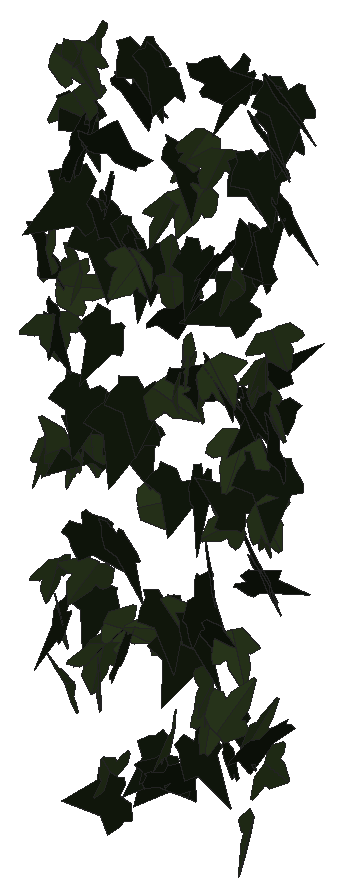
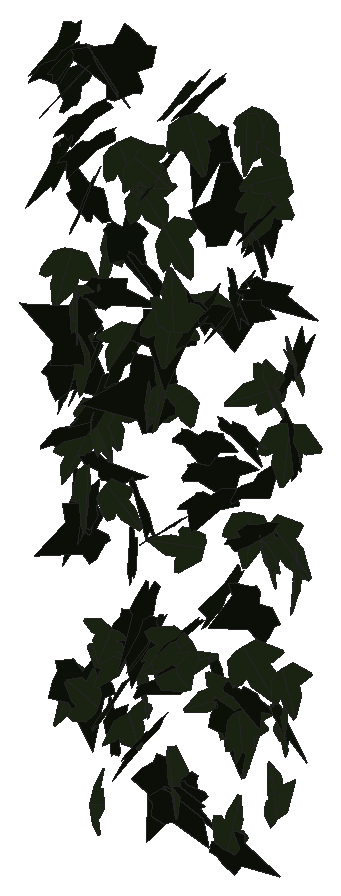
# SketchUp Ruby script. Lengths in inches.
U = 1.inch
M = Sketchup.active_model
def pt(a) = Geom::Point3d.new(a.map { |v| v * U })
def face(e, loops, mat)
  f = e.add_face(loops[0].map { |a| pt(a) })
  loops[1..].each { |l| e.add_face(l.map { |a| pt(a) }).erase! }
  f.material = f.back_material = mat if mat
  f
end
# faces: each face lists its corners as indices into pts; further lists are holes
def faces(e, pts, list, mat = nil) = list.each { |f| face(e, (f[0].is_a?(Array) ? f : [f]).map { |l| l.map { |i| pts[i] } }, mat) }
# xy, xz, yz: faces in a plane at the given z, y or x. An outline is a flat list of corners, or four numbers for a rectangle; further outlines are holes
def ring(l) = l.size == 4 ? [[l[0], l[1]], [l[2], l[1]], [l[2], l[3]], [l[0], l[3]]] : l.each_slice(2).to_a
def flat(e, list, mat, &to3) = list.each { |f| face(e, (f[0].is_a?(Array) ? f : [f]).map { |l| ring(l).map { |u, v| to3.(u, v) } }, mat) }
def xy(e, z, list, mat = nil) = flat(e, list, mat) { |x, y| [x, y, z] }
def xz(e, y, list, mat = nil) = flat(e, list, mat) { |x, z| [x, y, z] }
def yz(e, x, list, mat = nil) = flat(e, list, mat) { |y, z| [x, y, z] }
def lines(e, pts, list) = list.each { |a, b| e.add_line(pt(pts[a]), pt(pts[b])) }
# prism: a flat outline (further loops are holes) pulled along v
def prism(e, loops, v, mat = nil)
  f = face(e, loops, mat); d = Geom::Vector3d.new(v.map { |x| x * U })
  f.pushpull(f.normal.samedirection?(d) ? d.length : -d.length)
end
def box(e, o, s, mat = nil) = prism(e, [[o, [o[0] + s[0], o[1], o[2]], [o[0] + s[0], o[1] + s[1], o[2]], [o[0], o[1] + s[1], o[2]]]], [0, 0, s[2]], mat)
def at(x, y, z, deg = 0) = Geom::Transformation.translation(pt([x, y, z])) * Geom::Transformation.rotation(ORIGIN, Z_AXIS, deg.degrees)
def axes(o, x, y, z) = Geom::Transformation.new([*x, 0, *y, 0, *z, 0, *pt(o).to_a, 1])
def part(name) = M.definitions.add(name)
# library, detail: a bought-in or finely detailed component or shape, given as its bounding box
def library(name, o, s) = part(name).tap { |d| box(d.entities, o, s) }
def detail(e, o, s) = box(e.add_group.entities, o, s)
def put(e, d, t, mat = nil) = e.add_instance(d, t).tap { |i| i.material = mat if mat }
def group(e, t, mat = nil) = e.add_group.tap { |g| g.transformation = t; g.material = mat if mat }.entities
root = M.entities
M.materials.add("efeu1").color = [18, 25, 13]
M.materials.add("efeu2").color = [43, 57, 29]
c1 = part("ivyleaf_9")
p = [[1.54,2.16,1.25],[1.36,2.04,1.19],[-0.21,0.99,0.68],[-0.71,1.11,0.82],[-0.85,0.86,0.67],[-0.8,0.17,0.21],
  [-0.9,-0.01,0.1],[-0.67,-0.16,-0.02],[-0.08,-0.08,-0.05],[-0.03,-0.6,-0.4],[0.65,-0.88,-0.66],[0.83,-0.6,-0.49],
  [1.29,-0.42,-0.43],[1.8125,-0.07,-0.26],[1.21,0.44,0.15]]
faces(c1.entities,p,[[0,1,2,3,4,5,6,7,8,9,10,11,12,13,14]],"efeu1")
c2 = part("ivyleaf_10")
p = [[0,0.5,-0.03],[-0.0625,2.02,-0.43],[-0.19,2.01,-0.46],[-0.54,1.05,-0.29],[-0.52,0.625,-0.18],[-0.83,0.76,-0.28],
  [-1.16,0.64,-0.33],[-1.15,0.33,-0.24],[-0.77,-0.39,0.02],[-0.3,-0.51,0.16],[0.04,-0.48,0.23],[-0.02,2.01,-0.4375],
  [-0.06,2.01,-0.43],[0.04,-0.49,0.23],[0.67,-0.49,0.14],[1.38,0.36,-0.2],[1.375,0.51,-0.24],[0.81,0.65,-0.19],
  [0.62,0.59,-0.15],[0.6,1.09,-0.28],[0.5,1.23,-0.31]]
faces(c2.entities,p,[[0,1,2,3,4,5,6,7,8,9,10],[11,12,0,13,14,15,16,17,18,19,20]],"efeu2")
put(root,c1,axes([556.96,126.85,213.5],[-0.04115,0.46001,0.83642],[-0.11422,0.82881,-0.46144],[-0.94771,-0.11987,0.0193]))
put(root,c2,axes([563.91,127.77,229.87],[0.04295,-0.99561,0.12288],[0.05249,-0.1206,-0.99543],[1.00179,0.049,0.04689]))
put(root,c2,axes([562.57,126.82,212.66],[0.29842,0.56117,-0.90359],[0.36551,0.82723,0.63446],[0.9989,-0.47034,0.03779]))
put(root,c1,axes([563.42,128.23,219.59],[-0.00074,-0.33269,1.07237],[0.43668,-0.98803,-0.30622],[1.0344,0.41687,0.13005]))
put(root,c1,axes([556.12,127.79,206.37],[-0.18509,-0.18046,-0.9132],[-0.73724,-0.54002,0.25614],[-0.56831,0.75932,-0.03487]))
put(root,c2,axes([554.31,127.5,241.82],[-1.02474,0.14394,-0.2906],[0.28612,-0.0521,-1.03473],[-0.15266,-1.06387,0.01136]))
put(root,c2,axes([555.28,127.78,213.03],[-0.45322,-0.9324,0.17488],[-0.04544,-0.17226,-1.03616],[0.94757,-0.45422,0.03396]))
put(root,c1,axes([551.96,128.43,230.85],[-0.09599,-0.54405,0.96814],[0.20635,-0.96357,-0.52102],[1.0912,0.13435,0.18369]))
put(root,c1,axes([558.13,128.39,241.92],[-0.10549,-0.86154,0.61105],[0.18313,-0.6197,-0.84213],[1.04024,0.02173,0.21022]))
put(root,c2,axes([561.73,127.32,229.05],[0.31502,0.84677,0.37219],[0.14771,0.34208,-0.9033],[-0.91309,0.34748,-0.01772]))
put(root,c2,axes([564.7,127.16,211.14],[-0.06467,-0.7813,-0.75993],[0.13916,0.74912,-0.78203],[1.081,-0.14318,0.05521]))
put(root,c2,axes([557.07,127.76,232.33],[0.90924,-0.05206,-0.47628],[-0.4752,0.03248,-0.91072],[0.06118,1.02592,0.00467]))
put(root,c1,axes([563.52,128.48,234.65],[-0.09725,-0.35412,0.97283],[-0.07663,-0.97197,-0.36147],[1.03244,-0.1055,0.0648]))
put(root,c2,axes([558.8,127.46,226.9],[-0.4961,-0.37935,-0.73161],[0.7217,0.21231,-0.59946],[0.39789,-0.85808,0.17512]))
put(root,c1,axes([556.53,128.1875,224.72],[-0.65603,-0.87187,-0.17445],[0.10966,0.1358,-1.0911],[0.88236,-0.6651,0.0059]))
put(root,c2,axes([554.79,128.13,211.92],[0.37628,-0.38277,0.77565],[0.65648,-0.42438,-0.52789],[0.56318,0.75041,0.09711]))
put(root,c1,axes([563.4,127.71,234.61],[-0.44422,0.38361,0.92445],[0.64946,-0.65908,0.58558],[0.76155,0.78584,0.03985]))
put(root,c1,axes([554.09,128.3,224.9],[-0.23015,-0.99245,0.12721],[-0.02988,-0.12366,-1.01878],[1.00012,-0.23208,-0.00116]))
put(root,c2,axes([560.25,128.13,236.59],[-0.45584,-0.70848,0.50873],[-0.08625,-0.53459,-0.82177],[0.86793,-0.42522,0.18553]))
put(root,c2,axes([555.53,128.26,207],[-0.15251,-0.70602,-0.60976],[-0.02381,-0.6147,0.7177],[-0.93258,0.13116,0.08139]))
put(root,c2,axes([553.34,127.74,222.29],[-0.62841,-0.13183,0.94599],[-0.92672,-0.18997,-0.64208],[0.23121,-1.11969,-0.00244]))
put(root,c1,axes([564.24,128.47,225.67],[-0.07422,-0.27151,1.00837],[0.08294,-1.00925,-0.26565],[1.04098,0.06105,0.09306]))
put(root,c1,axes([560.77,128.25,218.3],[-0.03714,0.01892,0.92509],[0.16725,-0.91044,0.02533],[0.91004,0.1681,0.0331]))
put(root,c1,axes([554.34,126.93,237.34],[-0.1579,0.36324,-1.00284],[-0.76071,0.67224,0.36327],[0.74762,0.76073,0.15783]))
put(root,c1,axes([555.83,128.14,218.61],[0.54822,-0.90912,0.265],[0.14478,-0.22214,-1.06159],[0.93583,0.56695,0.009]))
put(root,c1,axes([559.26,128.38,237.93],[0.26468,-0.96173,0.46345],[0.13628,-0.44313,-0.9974],[1.05883,0.29744,0.01253]))
put(root,c1,axes([561.17,128.36,228.1],[0.26521,-0.70377,0.63807],[0.28525,-0.57289,-0.75045],[0.90612,0.38634,0.04949]))
put(root,c1,axes([563.62,128.24,240.77],[0.47323,-0.6754,0.56397],[0.33323,-0.4551,-0.82464],[0.81437,0.5787,0.0097]))
put(root,c1,axes([563.26,127.54,228],[0.72881,-0.37273,-0.58808],[-0.51666,0.28116,-0.8185],[0.46672,0.89328,0.01224]))
put(root,c2,axes([564.69,127.67,231.62],[-0.60628,-0.74749,-0.29267],[0.20858,0.20748,-0.96199],[0.77517,-0.64046,0.02994]))
put(root,c1,axes([561.55,127.875,234.3],[-0.40553,0.79059,-0.42816],[0.18074,-0.38843,-0.88841],[-0.88073,-0.44374,0.01483]))
put(root,c1,axes([563.53,128.13,239.35],[0.05083,-0.96506,-0.23992],[0.00881,0.24066,-0.96617],[0.9944,0.0472,0.02083]))
put(root,c1,axes([557.15,128.1,242.55],[0.28565,-1.0189,-0.20422],[0.00259,0.21249,-1.05655],[1.03917,0.27955,0.05877]))
put(root,c1,axes([553.07,128.06,213.98],[-0.79451,0.38254,-0.44095],[0.40062,-0.18434,-0.88178],[-0.42458,-0.88978,-0.00689]))
put(root,c2,axes([564.125,127.49,222.92],[0.08424,0.91846,0.37096],[0.03967,0.36887,-0.9223],[-0.98976,0.09296,-0.00539]))
put(root,c2,axes([560.96,127.72,213.3],[0.71943,-0.66194,-0.52085],[-0.32633,0.41243,-0.9749],[0.77651,0.78661,0.07286]))
put(root,c2,axes([559.3125,128.41,228.77],[-0.42038,0.24619,-0.83192],[0.34213,-0.80248,-0.41036],[-0.79727,-0.47417,0.26255]))
put(root,c1,axes([553.96,128.42,234.27],[-0.97197,-0.29067,0.36021],[-0.34794,-0.09369,-1.01445],[0.30525,-1.03232,-0.00936]))
put(root,c1,axes([563.79,127.67,219.99],[0.8011,-0.12733,-0.47848],[-0.47631,0.0504,-0.81087],[0.13523,0.93175,-0.02153]))
put(root,c1,axes([555.26,128.25,236.91],[1.16197,0.04712,0.13204],[-0.13204,-0.00281,1.16293],[0.04714,-1.16945,0.00252]))
put(root,c2,axes([564.03,127.77,230.06],[0.27753,-0.94116,-0.40182],[-0.03605,0.40708,-0.97839],[1.02271,0.26975,0.07455]))
put(root,c2,axes([562.48,128.08,225.45],[1.05871,0.30675,-0.19017],[-0.18227,-0.05426,-1.10226],[-0.31151,1.07429,-0.00137]))
put(root,c1,axes([560.25,127.9,210.29],[0.53104,-0.81397,-0.44891],[-0.17305,0.42139,-0.96878],[0.9133,0.55313,0.07746]))
put(root,c1,axes([557.07,128.29,226.02],[-0.60219,-0.61477,-0.41336],[0.31879,0.26581,-0.85974],[0.66872,-0.68032,0.03762]))
put(root,c2,axes([552,127.98,230.5625],[0.8213,-0.66676,0.03168],[-0.00422,0.04505,1.05738],[-0.66749,-0.82067,0.0323]))
put(root,c2,axes([561.95,128.16,221.43],[-0.56678,0.00415,0.74017],[-0.70589,-0.28349,-0.53894],[0.22268,-0.8881,0.17549]))
put(root,c1,axes([554.26,127.9,218.65],[-0.07936,-0.03443,-0.9948],[0.7537,0.64979,-0.08262],[0.6502,-0.75743,-0.02565]))
put(root,c1,axes([563.87,127.72,211.84],[-0.05359,1.11353,-0.19815],[-0.01265,-0.19895,-1.11461],[-1.13096,-0.05054,0.02186]))
put(root,c1,axes([551.9,128.47,227.67],[0.08296,-0.19874,-1.04068],[1.05949,0.01867,0.08089],[0.00316,-1.04382,0.19959]))
put(root,c1,axes([562.7,127.99,222.3],[-0.28638,0.3559,0.81761],[-0.80241,0.27173,-0.39934],[-0.38896,-0.8226,0.22183]))
put(root,c1,axes([557.125,128.48,232.6],[-0.68031,-0.23476,-0.695],[0.70664,0.04481,-0.70683],[0.19698,-0.97152,0.13535]))
put(root,c1,axes([558.13,128.55,215.97],[0.14563,-1.01866,-0.0126],[-0.00212,0.01243,-1.02901],[1.01873,0.14565,-0.00034]))
put(root,c2,axes([562.34,128.82,206.54],[0.23114,-0.45617,0.968],[0.64244,-0.73284,-0.49876],[0.8558,0.67334,0.11297]))
put(root,c1,axes([563.89,128.62,227.57],[-0.09923,0.41129,-0.95314],[0.07181,-0.95247,-0.41847],[-1.0356,-0.10546,0.06231]))
put(root,c1,axes([558.89,127.63,208.53],[0.66064,0.78429,-0.03153],[-0.02649,-0.01891,-1.02542],[-0.78447,0.66112,0.00808]))
put(root,c2,axes([552.36,128.38,215.93],[-0.13703,-0.89487,0.15217],[0.00386,-0.15447,-0.9049],[0.90771,-0.13444,0.02683]))
put(root,c1,axes([560.88,127.97,242.35],[0.52466,-0.06465,0.98926],[0.98462,-0.0964,-0.5285],[0.11549,1.11562,0.01166]))
put(root,c2,axes([554.23,128.51,216.35],[-0.58443,-0.66081,0.51555],[-0.3443,-0.38374,-0.88217],[0.76414,-0.6783,-0.00317]))
put(root,c2,axes([552.05,127.89,221.61],[0.35329,-0.86472,-0.61308],[-0.04541,0.6333,-0.9194],[1.05903,0.31563,0.1651]))
put(root,c2,axes([552.1875,128.64,213.52],[0.19262,-0.27309,0.86289],[0.80434,-0.35283,-0.29121],[0.41496,0.81067,0.16394]))
put(root,c1,axes([558.33,128.4,208.17],[0.20273,0.38091,-0.79878],[-0.3916,-0.69626,-0.43141],[-0.79359,0.44087,0.00882]))
put(root,c2,axes([558.34,128.68,235.43],[-0.01819,-1.0076,0.41582],[-0.03428,-0.41514,-1.00746],[1.08949,-0.02988,-0.02475]))
put(root,c1,axes([559.89,128.62,233.46],[-0.75738,-0.18548,-0.58185],[0.58904,0.02278,-0.77401],[0.16118,-0.9548,0.09457]))
put(root,c2,axes([562.34,127.76,233.52],[0.13966,-0.75749,-0.81498],[-0.06329,0.81464,-0.76802],[1.11085,0.14165,0.05871]))
put(root,c1,axes([563.66,128.75,224.4],[-0.1714,-1.08547,-0.1402],[0.03643,0.13617,-1.09882],[1.09388,-0.17461,0.01463]))
put(root,c2,axes([553.36,128.45,221.91],[0.77331,-0.51798,0.01839],[0.01642,-0.00854,-0.93075],[0.51804,0.77348,0.00205]))
put(root,c1,axes([555.04,128.625,233.08],[-0.4878,-0.88386,-0.4176],[0.17964,0.3777,-1.00927],[0.9609,-0.51931,-0.02331]))
put(root,c1,axes([562.02,128.1,209.67],[0.20362,-0.3916,0.81944],[-0.28081,0.77149,0.43846],[-0.8637,-0.34315,0.05063]))
put(root,c1,axes([556.76,127.97,240.72],[0.88102,0.28104,-0.58194],[-0.56829,-0.13157,-0.92389],[-0.30771,1.04763,0.04009]))
put(root,c2,axes([554.43,128.26,222.69],[-0.91617,-0.23142,0.04825],[-0.04604,-0.01476,-0.94494],[0.23187,-0.91732,0.00303]))
put(root,c1,axes([559.5625,128.62,215.38],[0.56135,-0.8755,0.09688],[0.05414,-0.08038,-1.04001],[0.87918,0.56395,0.00218]))
put(root,c2,axes([561.03,128.6,238.54],[-0.42852,-0.82164,0.33797],[-0.16099,-0.29721,-0.92666],[0.87373,-0.45773,-0.00498]))
put(root,c1,axes([554.13,129,222.53],[-0.66689,-0.54566,0.43347],[-0.30315,-0.31309,-0.8605],[0.62749,-0.73118,0.04497]))
put(root,c2,axes([552.3125,128.29,227.7],[-0.79347,-0.70618,-0.08184],[0.06106,0.05449,-1.06221],[0.70828,-0.79582,-0.00011]))
put(root,c1,axes([563.2,127.84,219.19],[0.7574,0.30109,0.46491],[0.4054,0.23533,-0.81285],[-0.37743,0.85699,0.05987]))
put(root,c2,axes([558.25,129.02,214.58],[0.03717,0.29167,1.04358],[-0.44389,-0.94845,0.28089],[0.98847,-0.43689,0.0869]))
put(root,c1,axes([553.43,128.58,236.01],[-0.10786,0.66897,0.83861],[0.12026,-0.82998,0.67756],[1.06598,0.16133,0.00842]))
put(root,c2,axes([559.46,128.79,226.48],[-0.61943,0.18058,0.88303],[0.81607,-0.34245,0.64249],[0.38259,1.02282,0.05921]))
put(root,c1,axes([557.93,128.71,208.57],[-0.90536,-0.01366,-0.00853],[0.00854,-0.00012,-0.90546],[0.01365,-0.9054,0.00025]))
put(root,c1,axes([556.55,129.19,232],[0.15202,-0.85598,0.74744],[0.2793,-0.70283,-0.86169],[1.10153,0.29633,0.11534]))
put(root,c1,axes([559,128.0625,230.72],[0.2379,0.92417,-0.18748],[-0.0666,-0.1764,-0.95409],[-0.94064,0.24623,0.02014]))
put(root,c2,axes([563.24,128.7,227.95],[-0.67483,0.42661,-0.8087],[0.63847,-0.49959,-0.79633],[-0.65448,-0.92725,0.05699]))
put(root,c1,axes([558.8,129.12,213.95],[-0.37855,-0.89782,0.18594],[-0.04726,-0.18179,-0.974],[0.91566,-0.38056,0.02661]))
put(root,c2,axes([554.43,128.32,242.07],[0.01777,-0.94548,-0.37206],[-0.01894,0.37174,-0.94558],[1.01587,0.02347,-0.01112]))
put(root,c2,axes([559.77,128.9,238.6875],[0.29669,0.72316,-0.64219],[-0.46401,-0.48294,-0.7582],[-0.84857,0.51692,0.19006]))
put(root,c2,axes([552.32,128.99,209.92],[-0.70394,0.04576,0.86687],[0.79463,-0.41533,0.6672],[0.34946,1.03658,0.22906]))
put(root,c2,axes([553.5,128.32,238.92],[-0.52945,-0.8289,-0.45128],[0.25109,0.37508,-0.98352],[0.90977,-0.5859,0.00882]))
put(root,c1,axes([562.1,128.91,242.72],[-0.87324,0.16856,-0.48498],[0.45597,-0.18524,-0.88541],[-0.23601,-0.98155,0.08382]))
put(root,c1,axes([561.99,129.07,231.71],[-0.78993,-0.22021,0.56102],[-0.5372,-0.16203,-0.81999],[0.27322,-0.95524,0.00976]))
put(root,c1,axes([559.39,128.0625,227.16],[0.78505,0.19406,0.84294],[0.81884,0.20012,-0.80868],[-0.27875,1.13437,-0.00154]))
put(root,c2,axes([554.57,128.62,213.01],[-0.05485,-1.09654,-0.1535],[-0.00368,0.15387,-1.09785],[1.10723,-0.05381,-0.01125]))
put(root,c1,axes([555.28,128.23,213.21],[-0.14356,0.93492,0.00845],[-0.00437,0.00788,-0.94587],[-0.93495,-0.14359,0.00312]))
put(root,c1,axes([553.21,128.84,238.28],[0.33426,-0.93672,-0.22513],[-0.06339,0.2164,-0.99449],[0.96131,0.33998,0.01271]))
put(root,c2,axes([558.03,128.52,215.55],[-0.79556,-0.0538,-0.84648],[0.84668,0.01896,-0.79695],[0.05067,-1.16151,0.0262]))
put(root,c1,axes([559.75,128.98,222.35],[-0.65044,0.07003,-0.87715],[0.87585,-0.05353,-0.65375],[-0.08475,-1.09068,-0.02424]))
put(root,c1,axes([562.65,128.81,238.59],[0.14707,-0.93718,-0.37445],[0.04172,0.38373,-0.94401],[1.00835,0.12081,0.09367]))
put(root,c1,axes([560.22,128.375,215.85],[0.67736,0.38931,-0.48773],[-0.45193,-0.19038,-0.7796],[-0.43036,0.81268,0.05101]))
put(root,c1,axes([558.24,129.34,221.52],[-0.22447,-0.89091,0.28966],[0.1766,-0.33276,-0.88662],[0.92003,-0.15349,0.24086]))
put(root,c2,axes([552.57,128.51,240.33],[0.45664,-0.13516,0.8889],[0.842,0.41397,-0.36959],[-0.31537,0.90956,0.30031]))
put(root,c2,axes([558.37,128.53,209.89],[0.3628,-1.02114,-0.46893],[-0.16,0.4408,-1.08367],[1.11222,0.3965,-0.00293]))
put(root,c2,axes([559.34,127.96,227.01],[0.20076,-0.24107,1.13152],[-0.64654,0.92898,0.31263],[-0.95939,-0.67649,0.02609]))
put(root,c1,axes([554.56,128.68,233.88],[0.73482,-0.73887,-0.29181],[-0.19333,0.21923,-1.04192],[0.77053,0.75964,0.01686]))
put(root,c2,axes([563.31,128.33,221.83],[-0.75972,0.51567,0.63935],[-0.56123,0.31001,-0.91693],[-0.59975,-0.94331,0.04816]))
put(root,c1,axes([560.08,128.14,217.16],[0.34249,-0.29062,-1.08098],[-0.8026,0.72423,-0.449],[0.78026,0.87253,0.01264]))
put(root,c1,axes([554.19,129.0625,214.97],[-0.77884,-0.29801,-0.42666],[0.41518,0.10725,-0.8328],[0.3138,-0.88154,0.04291]))
put(root,c1,axes([556.0625,128.85,223.7],[-0.09575,-0.78817,-0.51115],[0.12015,0.49931,-0.79241],[0.93169,-0.1454,0.04966]))
put(root,c1,axes([561.23,128.93,212],[0.55492,-0.81786,-0.1043],[-0.06185,0.08407,-0.98834],[0.82216,0.55834,-0.00396]))
put(root,c2,axes([560.32,128.99,211.5],[0.28387,0.96285,-0.40093],[-0.10626,-0.38666,-1.0038],[-1.03756,0.30303,-0.00689]))
put(root,c1,axes([563.71,129.49,240.78],[-0.00848,-0.90775,0.46827],[0.08584,-0.46727,-0.90424],[1.0178,0.03184,0.08017]))
put(root,c1,axes([563.72,128.88,242.83],[0.82586,-0.62141,0.09302],[0.07392,-0.05648,-1.03353],[0.62397,0.82916,-0.00069]))
put(root,c1,axes([563.34,128.26,228.77],[0.37789,0.94149,-0.40292],[0.08275,0.4,1.01228],[1.02074,-0.38098,0.0671]))
put(root,c1,axes([564.14,128.71,237.35],[0.88326,-0.52878,-0.31119],[-0.26867,0.15706,-1.02944],[0.55161,0.92321,-0.00311]))
put(root,c2,axes([561.9,129.1875,225.26],[0.30837,-0.88463,0.29249],[0.08529,-0.27999,-0.93678],[0.92782,0.31976,-0.0111]))
put(root,c1,axes([564.03,129.34,242.37],[-0.09286,-1.03662,-0.03036],[0.00371,0.03014,-1.04077],[1.03706,-0.09292,0.00101]))
put(root,c2,axes([557.34,128.43,220.64],[0.19942,0.03521,-0.93105],[0.81396,0.45674,0.19161],[0.45339,-0.83547,0.06552]))
put(root,c2,axes([558.34,128.81,231.41],[-0.92374,-0.38282,0.00582],[-0.00548,-0.00197,-0.99992],[0.38283,-0.92375,-0.00028]))
put(root,c2,axes([562.89,128.51,211.18],[0.14908,-0.77037,0.57617],[-0.08913,0.56948,0.78449],[-0.95786,-0.17289,0.01668]))
put(root,c2,axes([561.41,128.91,215.18],[0.8608,0.16369,0.43784],[0.43286,0.06714,-0.87612],[-0.17642,0.96341,-0.01333]))
put(root,c2,axes([553.1875,128.21,229.7],[0.06341,0.16377,1.02197],[0.41052,0.93592,-0.17545],[-0.95011,0.41532,-0.0076]))
put(root,c1,axes([554.49,129.23,227.8],[-0.87538,-0.18721,-0.30549],[0.30584,0.02968,-0.89456],[0.18664,-0.92668,0.03307]))
put(root,c2,axes([557.89,129.01,231.85],[-1.01666,-0.16054,0.19002],[0.18964,0.01721,1.02918],[-0.16099,1.03412,0.01237]))
put(root,c2,axes([553.23,128.54,230.34],[0.31979,-0.35302,-0.91849],[-0.6626,0.63674,-0.47543],[0.72746,0.73515,-0.02927]))
put(root,c1,axes([561.61,128.95,226.65],[0.79127,-0.62138,0.00652],[0.00352,-0.00608,-1.00609],[0.6214,0.79128,-0.0026]))
put(root,c2,axes([555.51,128.4,214.04],[0.2014,0.20067,0.88907],[0.52391,0.71958,-0.28109],[-0.74581,0.55966,0.04263]))
put(root,c1,axes([554.53,129.27,234.58],[-0.54585,0.22324,-0.80192],[0.74162,-0.30508,-0.58974],[-0.37803,-0.92084,0.00097]))
put(root,c2,axes([557.15,128.94,241.27],[-0.8593,-0.30151,0.46438],[-0.43748,-0.15578,-0.91066],[0.33937,-0.96425,0.00191]))
